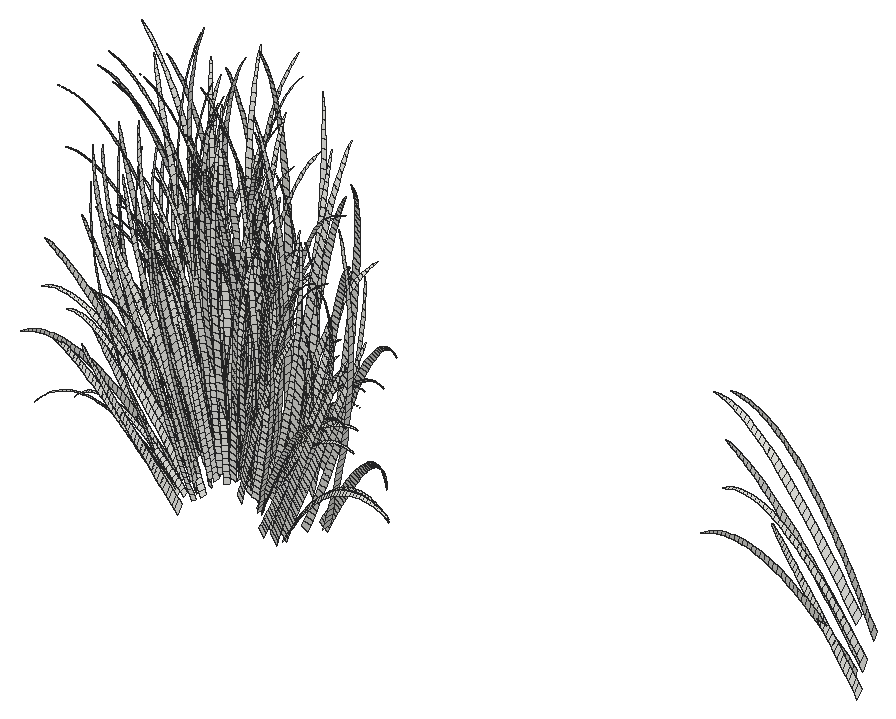
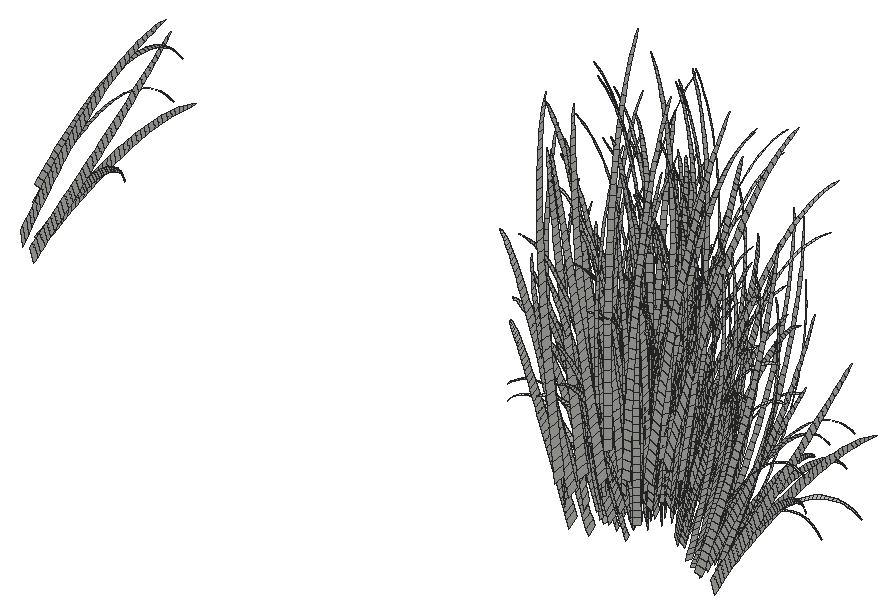
# SketchUp Ruby script. Lengths in inches.
U = 1.inch
M = Sketchup.active_model
def pt(a) = Geom::Point3d.new(a.map { |v| v * U })
def face(e, loops, mat)
  f = e.add_face(loops[0].map { |a| pt(a) })
  loops[1..].each { |l| e.add_face(l.map { |a| pt(a) }).erase! }
  f.material = f.back_material = mat if mat
  f
end
# faces: each face lists its corners as indices into pts; further lists are holes
def faces(e, pts, list, mat = nil) = list.each { |f| face(e, (f[0].is_a?(Array) ? f : [f]).map { |l| l.map { |i| pts[i] } }, mat) }
# xy, xz, yz: faces in a plane at the given z, y or x. An outline is a flat list of corners, or four numbers for a rectangle; further outlines are holes
def ring(l) = l.size == 4 ? [[l[0], l[1]], [l[2], l[1]], [l[2], l[3]], [l[0], l[3]]] : l.each_slice(2).to_a
def flat(e, list, mat, &to3) = list.each { |f| face(e, (f[0].is_a?(Array) ? f : [f]).map { |l| ring(l).map { |u, v| to3.(u, v) } }, mat) }
def xy(e, z, list, mat = nil) = flat(e, list, mat) { |x, y| [x, y, z] }
def xz(e, y, list, mat = nil) = flat(e, list, mat) { |x, z| [x, y, z] }
def yz(e, x, list, mat = nil) = flat(e, list, mat) { |y, z| [x, y, z] }
def lines(e, pts, list) = list.each { |a, b| e.add_line(pt(pts[a]), pt(pts[b])) }
# prism: a flat outline (further loops are holes) pulled along v
def prism(e, loops, v, mat = nil)
  f = face(e, loops, mat); d = Geom::Vector3d.new(v.map { |x| x * U })
  f.pushpull(f.normal.samedirection?(d) ? d.length : -d.length)
end
def box(e, o, s, mat = nil) = prism(e, [[o, [o[0] + s[0], o[1], o[2]], [o[0] + s[0], o[1] + s[1], o[2]], [o[0], o[1] + s[1], o[2]]]], [0, 0, s[2]], mat)
def at(x, y, z, deg = 0) = Geom::Transformation.translation(pt([x, y, z])) * Geom::Transformation.rotation(ORIGIN, Z_AXIS, deg.degrees)
def axes(o, x, y, z) = Geom::Transformation.new([*x, 0, *y, 0, *z, 0, *pt(o).to_a, 1])
def part(name) = M.definitions.add(name)
# library, detail: a bought-in or finely detailed component or shape, given as its bounding box
def library(name, o, s) = part(name).tap { |d| box(d.entities, o, s) }
def detail(e, o, s) = box(e.add_group.entities, o, s)
def put(e, d, t, mat = nil) = e.add_instance(d, t).tap { |i| i.material = mat if mat }
def group(e, t, mat = nil) = e.add_group.tap { |g| g.transformation = t; g.material = mat if mat }.entities
root = M.entities
c1 = part("fur_instance\#8")
p = [[-0.25,1.49,0.03],[0.25,-1.49,-0.03],[0.44,-1.47,1.51],[-0.05,1.47,1.57],[0.65,-1.44,3.05],[0.16,1.45,3.11],
  [0.86,-1.42,4.59],[0.38,1.44,4.65],[1.1,-1.39,6.13],[0.62,1.43,6.18],[1.34,-1.35,7.66],[0.875,1.42,7.72],
  [1.6,-1.32,9.19],[1.14,1.41,9.25],[1.88,-1.28,10.72],[1.43,1.41,10.78],[2.18,-1.24,12.25],[1.73,1.41,12.3],
  [2.49,-1.19,13.77],[2.05,1.41,13.82],[2.83,-1.15,15.29],[2.4,1.41,15.34],[3.18,-1.09,16.8],[2.76,1.42,16.85],
  [3.56,-1.03,18.31],[3.14,1.43,18.35],[3.96,-0.97,19.81],[3.55,1.44,19.85],[4.38,-0.91,21.3],[3.99,1.46,21.35],
  [4.84,-0.83,22.78],[4.45,1.48,22.83],[5.32,-0.76,24.26],[4.93,1.51,24.31],[5.82,-0.67,25.73],[5.45,1.54,25.77],
  [6.36,-0.59,27.18],[6,1.57,27.23],[6.93,-0.49,28.625],[6.58,1.61,28.67],[7.54,-0.39,30.05],[7.19,1.66,30.1],
  [8.18,-0.28,31.47],[7.84,1.71,31.51],[8.85,-0.16,32.86],[8.53,1.77,32.9],[9.57,-0.04,34.24],[9.25,1.83,34.27],
  [10.32,0.09,35.59],[10.02,1.9,35.625],[11.12,0.23,36.92],[10.82,1.97,36.95],[11.95,0.38,38.22],[11.67,2.06,38.25],
  [12.84,0.54,39.49],[12.57,2.14,39.52],[13.76,0.71,40.73],[13.51,2.24,40.76],[14.73,0.89,41.93],[14.49,2.34,41.95],
  [15.75,1.08,43.09],[15.52,2.45,43.11],[16.82,1.28,44.2],[16.6,2.5625,44.23],[17.93,1.5,45.27],[17.73,2.68,45.29],
  [19.08,1.73,46.28],[18.9,2.81,46.3],[20.29,1.97,47.24],[20.125,2.93,47.26],[21.53,2.22,48.13],[21.39,3.0625,48.15],
  [22.82,2.5,48.96],[22.7,3.1875,48.98],[24.14,2.8125,49.72],[24.06,3.3,49.73],[25.48,3.27,50.41]]
faces(c1.entities,p,[[0,1,2,3],[3,2,4,5],[5,4,6,7],[7,6,8,9],[9,8,10,11],[11,10,12,13],[13,12,14,15],[15,14,16,17],
  [17,16,18,19],[19,18,20,21],[21,20,22,23],[23,22,24,25],[25,24,26,27],[27,26,28,29],[29,28,30,31],[31,30,32,33],
  [33,32,34,35],[35,34,36,37],[37,36,38,39],[39,38,40,41],[41,40,42,43],[43,42,44,45],[45,44,46,47],[47,46,48,49],
  [49,48,50,51],[51,50,52,53],[53,52,54,55],[55,54,56,57],[57,56,58,59],[59,58,60,61],[61,60,62,63],[63,62,64,65],
  [65,64,66,67],[67,66,68,69],[69,68,70,71],[71,70,72,73],[73,72,74,75],[75,74,76]])
put(root,c1,axes([95.76,70.05,-3.04],[0.01897,-0.21218,0.0586],[0.13531,-0.01729,0.38322],[-0.17657,-0.01268,0.31544]))
put(root,c1,axes([96.34,68.3125,-2.78],[-0.03242,-0.16161,-0.19656],[0.13271,-0.12456,0.32589],[-0.17032,-0.04313,0.30667]))
put(root,c1,axes([97.72,67.32,-0.53],[-0.17146,0.07712,-0.27655],[0.00216,-0.17859,-0.14821],[-0.13359,-0.07259,0.37194]))
put(root,c1,axes([97.38,67.44,-3.66],[-0.07927,0.1771,-0.13212],[-0.09456,-0.05104,-0.31736],[-0.15384,-0.03896,0.27701]))
put(root,c1,axes([97.58,67.0625,-2.9],[-0.11039,-0.00414,-0.3495],[0.07669,-0.1786,0.00651],[-0.14786,-0.06719,0.2791]))
put(root,c1,axes([98.16,65.8125,-2.88],[-0.13594,0.15084,-0.11164],[-0.0609,-0.07291,-0.33491],[-0.13519,-0.09407,0.27953]))
put(root,c1,axes([95.88,69.58,-2.68],[0.13391,-0.00422,0.37894],[-0.02725,0.21287,-0.08205],[-0.17659,-0.01268,0.31548]))
put(root,c1,axes([98.56,66.53,-1.61],[-0.14992,0.10635,-0.20855],[-0.03569,-0.13875,-0.18978],[-0.12006,-0.06524,0.33426]))
put(root,c1,axes([98.55,67.96,-1.74],[-0.13947,0.07457,-0.26376],[-0.03048,-0.16347,-0.05841],[-0.12421,-0.01975,0.3263]))
put(root,c1,axes([98.58,66.7,-3.14],[-0.11214,0.07357,-0.29467],[-0.00419,-0.1506,-0.10442],[-0.13991,-0.03543,0.25192]))
put(root,c1,axes([97.64,70.26,4.84],[-0.16722,-0.14584,-0.14657],[0.18274,-0.19209,0.09427],[-0.0816,-0.06233,0.55718]))
put(root,c1,axes([96.18,71.21,-1.63],[0.10956,-0.18152,0.25882],[0.13509,0.11782,0.19082],[-0.14519,0.00192,0.39222]))
put(root,c1,axes([97.17,69.17,-2.25],[0.07012,-0.18381,0.20265],[0.10518,0.07075,0.29594],[-0.16336,-0.01173,0.29184]))
put(root,c1,axes([97.06,66.95,-2.91],[0.11177,0.01694,0.37048],[-0.08915,0.18926,-0.03147],[-0.15727,-0.07147,0.29687]))
put(root,c1,axes([97.58,67.58,-2.4],[0.07273,0.09595,0.27862],[-0.10249,0.16133,-0.212],[-0.15668,-0.03967,0.28211]))
put(root,c1,axes([96.1,68.47,-1.64],[0.16226,-0.13696,0.26442],[0.06401,0.16282,0.19515],[-0.14822,-0.05035,0.39313]))
put(root,c1,axes([98.9375,68.57,3.38],[-0.19486,-0.07064,-0.15993],[0.11436,-0.20339,0.01183],[-0.07048,-0.06892,0.50496]))
put(root,c1,axes([99.14,65.35,-3.56],[-0.09839,0.14314,-0.01192],[-0.08354,-0.02419,-0.30566],[-0.11714,-0.08151,0.24221]))
put(root,c1,axes([98.54,68.2,-3.06],[-0.01321,-0.17005,0.06481],[0.1141,-0.02557,0.30569],[-0.13946,0.01456,0.25678]))
put(root,c1,axes([99.65,69.16,1.2],[-0.18243,0.01895,-0.19563],[-0.00133,-0.1948,0.08688],[-0.09334,0.00298,0.40574]))
put(root,c1,axes([99.52,67.88,-0.75],[-0.16023,0.03354,-0.19126],[-0.00898,-0.17162,0.02853],[-0.08895,-0.01176,0.36236]))
put(root,c1,axes([99.47,66.625,0.58],[-0.1494,0.14445,-0.05993],[-0.10862,-0.10225,-0.21391],[-0.08642,-0.08137,0.39881]))
put(root,c1,axes([96.96,68.125,-0.75],[0.16036,-0.12824,0.26431],[0.05712,0.1633,0.18167],[-0.14465,-0.04914,0.38366]))
put(root,c1,axes([97.38,68.18,-1.53],[0.12489,0.06673,0.27563],[-0.09958,0.18305,-0.12082],[-0.13573,-0.04611,0.36]))
put(root,c1,axes([99.77,66.73,-0.91],[-0.15052,-0.00251,-0.18515],[0.03159,-0.16716,0.03488],[-0.08794,-0.02622,0.34898]))
put(root,c1,axes([99.5,68.69,-0.2],[-0.10618,-0.13262,-0.04878],[0.13367,-0.1263,0.19427],[-0.08735,0.00279,0.37967]))
put(root,c1,axes([98.35,68.18,-3.57],[0.10833,0.05099,0.24664],[-0.03776,0.16401,-0.19126],[-0.1393,0.01454,0.25647]))
put(root,c1,axes([99.47,70.78,6.02],[-0.09372,-0.20637,-0.07363],[0.22677,-0.12712,0.15354],[-0.08199,-0.04812,0.55353]))
put(root,c1,axes([97.89,69.19,-1.1],[0.15491,-0.05585,0.29054],[0.02871,0.18789,-0.02061],[-0.13151,0.00174,0.35528]))
put(root,c1,axes([100.5,67.92,0.34],[-0.13836,0.10656,-0.19014],[-0.08729,-0.13946,-0.02631],[-0.08371,0.00267,0.36384]))
put(root,c1,axes([99.375,66.87,-1.86],[0.03066,0.14936,0.05869],[-0.12804,0.07175,-0.24213],[-0.11455,-0.01821,0.30092]))
put(root,c1,axes([99.75,66.9375,2.03],[-0.03053,0.18634,0.11663],[-0.19498,0.03215,-0.20672],[-0.09234,-0.08694,0.42611]))
put(root,c1,axes([99.99,66.09,0.62],[-0.076,0.1669,0.09562],[-0.17144,-0.01335,-0.19918],[-0.07397,-0.09509,0.39348]))
put(root,c1,axes([100.3125,67.9,0.96],[-0.14595,-0.08896,-0.08701],[0.11069,-0.159,0.08949],[-0.05969,-0.02587,0.41282]))
put(root,c1,axes([100.32,66.87,1.13],[-0.13003,0.1505,-0.04051],[-0.13515,-0.09639,-0.12681],[-0.0585,-0.05721,0.41915]))
put(root,c1,axes([100.31,69.73,4.93],[-0.20007,-0.1011,-0.05198],[0.13259,-0.20105,0.02025],[-0.03025,-0.05245,0.53866]))
put(root,c1,axes([100.8125,69.61,6.05],[-0.23914,-0.05106,-0.06078],[0.08551,-0.22855,-0.0252],[-0.02809,-0.06875,0.5682]))
put(root,c1,axes([99.25,67.93,-3.57],[0.06974,-0.11239,0.27242],[0.09117,0.10684,0.0892],[-0.12045,0.03482,0.23783]))
put(root,c1,axes([98.43,69.49,-1.98],[0.12819,-0.10555,0.27193],[0.08655,0.15023,0.02614],[-0.11644,0.02211,0.33646]))
put(root,c1,axes([99.42,66.64,-3.27],[0.09888,-0.02928,0.28041],[-0.00291,0.15131,-0.01175],[-0.12783,-0.00918,0.22836]))
put(root,c1,axes([99.94,68.41,-1.64],[-0.01787,-0.16163,0.13786],[0.14541,-0.01364,0.20157],[-0.09392,0.03632,0.30351]))
put(root,c1,axes([100.86,66.9,0.16],[-0.15295,0.08658,-0.10984],[-0.06653,-0.14152,-0.02919],[-0.05435,-0.02356,0.3759]))
put(root,c1,axes([100.52,68.36,-1.61],[-0.08732,-0.12975,0.07004],[0.12156,-0.08169,0.22443],[-0.07712,0.04857,0.29461]))
put(root,c1,axes([101.34,69.47,6.1],[-0.24023,0.10194,-0.01182],[-0.08393,-0.20819,-0.06775],[-0.02132,-0.07588,0.56748]))
put(root,c1,axes([99.06,66.95,-1.92],[0.13512,-0.04534,0.25565],[0.00767,0.16418,0.01521],[-0.11775,-0.01872,0.30933]))
put(root,c1,axes([101.21,66.88,0.11],[-0.16155,0.04363,-0.11105],[-0.02173,-0.15615,0.00187],[-0.05311,-0.02302,0.36735]))
put(root,c1,axes([101.125,68.14,0.01],[-0.13763,-0.08778,-0.02445],[0.09224,-0.14199,0.18002],[-0.06167,0.02548,0.35158]))
put(root,c1,axes([100.82,67.91,4.45],[-0.11071,0.19643,0.08485],[-0.20741,-0.05916,-0.14436],[-0.04649,-0.10158,0.50968]))
put(root,c1,axes([99.14,67.375,0.375],[0.12398,0.09622,0.18511],[-0.12468,0.16008,-0.11198],[-0.09878,-0.04719,0.39625]))
put(root,c1,axes([101.45,67.29,0.93],[-0.15275,-0.06369,-0.07605],[0.08272,-0.1606,0.08732],[-0.05298,-0.01559,0.38969]))
put(root,c1,axes([101.29,66.44,0.1],[-0.12167,0.12231,-0.08026],[-0.10576,-0.10199,-0.07795],[-0.05387,-0.03162,0.36369]))
put(root,c1,axes([99.79,67.73,0.52],[0.1073,0.11537,0.13468],[-0.12896,0.14123,-0.15523],[-0.09593,-0.0286,0.38067]))
put(root,c1,axes([101.6875,66.98,-0.06],[-0.15222,0.06371,-0.10078],[-0.04912,-0.14483,0.02613],[-0.04368,-0.00705,0.35627]))
put(root,c1,axes([101.84,66.57,1.76],[-0.18454,0.07316,-0.01839],[-0.05778,-0.16138,-0.04792],[-0.01906,-0.05522,0.43193]))
put(root,c1,axes([100.54,71.5625,4.7],[-0.03022,-0.22611,0.09029],[0.23429,-0.05028,0.11994],[-0.05481,-0.00145,0.5217]))
put(root,c1,axes([100.03,65.9,0.83],[0.08886,0.11953,0.22309],[-0.17307,0.12603,-0.0526],[-0.07674,-0.09865,0.40821]))
put(root,c1,axes([101.95,69.69,5.24],[-0.19122,-0.11806,-0.01455],[0.14538,-0.19433,0.04316],[-0.02276,-0.03764,0.53822]))
put(root,c1,axes([100.95,68.76,1.41],[-0.07059,-0.16734,0.04684],[0.17777,-0.08469,0.11217],[-0.04438,-0.00118,0.42241]))
put(root,c1,axes([102.04,67.4,0.8],[-0.1632,-0.04584,-0.02491],[0.06111,-0.16287,0.10545],[-0.03205,0.00396,0.38155]))
put(root,c1,axes([101.26,67.78,0.43],[-0.07809,-0.14325,0.0107],[0.15359,-0.09235,0.11164],[-0.04706,-0.00759,0.38378]))
put(root,c1,axes([102.12,68.24,1.7],[-0.18597,0.0618,-0.02273],[-0.04748,-0.17087,0.02426],[-0.01189,-0.02692,0.4292]))
put(root,c1,axes([100.38,67.35,-2.1],[0.12505,0.02128,0.17693],[-0.02026,0.14885,-0.13694],[-0.09536,0.01811,0.27556]))
put(root,c1,axes([98.5,70.37,4.92],[0.23978,-0.07082,0.15768],[0.03022,0.22441,0.06362],[-0.07961,-0.06081,0.54364]))
put(root,c1,axes([101.25,68.31,3.06],[-0.04674,0.1979,-0.00041],[-0.20698,-0.02041,-0.04932],[-0.02674,-0.04637,0.47621]))
put(root,c1,axes([98.9,68.09,4.41],[0.21026,0.07749,0.17035],[-0.13208,0.20951,0.0486],[-0.06062,-0.09852,0.54406]))
put(root,c1,axes([99.26,69.1,2.46],[0.19711,0.03834,0.13931],[-0.07116,0.20343,-0.04176],[-0.07003,-0.0411,0.47276]))
put(root,c1,axes([100.61,67.91,-0.74],[0.08378,-0.14307,0.16626],[0.13275,0.07958,0.06416],[-0.07048,0.0146,0.34149]))
put(root,c1,axes([102.4,65.47,-0.05],[-0.14611,0.07417,-0.01085],[-0.0636,-0.12579,-0.04088],[-0.01571,-0.04551,0.35595]))
put(root,c1,axes([101.92,65.52,-0.11],[-0.03907,0.14419,0.04289],[-0.15068,-0.00691,-0.10234],[-0.04404,-0.05511,0.34471]))
put(root,c1,axes([102.72,66.39,1.99],[-0.18895,0.06999,0.02245],[-0.05996,-0.16418,-0.04942],[-0.00199,-0.06326,0.44045]))
put(root,c1,axes([101.76,68.33,4.43],[-0.07149,0.20688,0.05021],[-0.22153,-0.04139,-0.03916],[-0.01557,-0.07173,0.51835]))
put(root,c1,axes([102.36,67.78,-0.98],[-0.12985,-0.07677,0.07158],[0.09092,-0.12597,0.14453],[-0.01646,0.03757,0.31821]))
put(root,c1,axes([101.85,66.36,0.1],[0.0007,0.15498,-0.03624],[-0.15701,0.01919,-0.0982],[-0.04789,-0.01409,0.35225]))
put(root,c1,axes([99.64,69.85,3.34],[0.21533,-0.00022,0.14201],[-0.02985,0.21622,-0.04212],[-0.07083,-0.0307,0.48991]))
put(root,c1,axes([101.76,69.9,1.31],[-0.05762,-0.17661,0.09378],[0.18885,-0.07013,0.07584],[-0.02585,0.00825,0.42914]))
put(root,c1,axes([102.47,66.12,1.29],[-0.11204,0.14362,0.03398],[-0.14775,-0.08605,-0.03808],[-0.00899,-0.05843,0.41243]))
put(root,c1,axes([101.42,66.88,0.34],[0.07256,0.13813,0.01061],[-0.14853,0.08916,-0.10968],[-0.05042,-0.01484,0.37084]))
put(root,c1,axes([103.28,68.28,2.5],[-0.20122,0.04978,0.02765],[-0.03696,-0.18587,0.02525],[0.00919,-0.0352,0.4569]))
put(root,c1,axes([102.08,69.16,2.61],[-0.07053,-0.17965,0.10788],[0.19435,-0.08267,0.06265],[-0.01549,0.01046,0.44704]))
put(root,c1,axes([102.6875,67,0.08],[-0.12044,0.11617,-0.06507],[-0.11184,-0.10532,0.07409],[-0.00291,0.00808,0.35453]))
put(root,c1,axes([101.09,66.82,1.47],[0.1306,0.09776,0.12408],[-0.13059,0.14634,-0.04229],[-0.05761,-0.05634,0.41276]))
put(root,c1,axes([102.94,67,0.32],[-0.14146,0.09732,-0.03277],[-0.08974,-0.12702,0.09515],[0.00654,0.00629,0.36155]))
put(root,c1,axes([102.26,66.14,1.84],[-0.02865,0.1632,0.13083],[-0.19416,0.00105,-0.04665],[-0.01776,-0.09378,0.4187]))
put(root,c1,axes([100.21,68.21,3.96],[0.21896,0.00722,0.14738],[-0.05367,0.20894,0.06409],[-0.06377,-0.07981,0.49923]))
put(root,c1,axes([102.14,66.79,0.41],[-0.005,0.15882,-0.01867],[-0.16818,0.01184,-0.02587],[-0.01594,-0.02637,0.37698]))
put(root,c1,axes([103.12,68.37,-1.29],[-0.15178,-0.03817,0.09021],[0.05761,-0.14672,0.13772],[0.01323,0.03497,0.32535]))
put(root,c1,axes([103.09,68.04,-0.72],[-0.14817,-0.05096,0.10268],[0.07099,-0.14472,0.13123],[0.01339,0.03539,0.32926]))
put(root,c1,axes([102.65,65.7,0.44],[-0.04364,0.1509,0.04181],[-0.16335,-0.02313,-0.02043],[-0.0082,-0.05328,0.37608]))
put(root,c1,axes([101.25,66.81,1.18],[0.16328,0.03799,0.12354],[-0.06943,0.16853,-0.0179],[-0.05845,-0.04464,0.39911]))
put(root,c1,axes([102.84,68.17,0.11],[-0.0829,-0.13844,0.09301],[0.15279,-0.09132,0.04718],[-0.00308,0.00854,0.37496]))
put(root,c1,axes([101.38,68.7,1.45],[0.11915,-0.15444,0.11959],[0.14734,0.10329,0.01409],[-0.04397,-0.00116,0.41847]))
put(root,c1,axes([100.86,68.36,1.08],[0.18469,-0.02182,0.1026],[0.00322,0.18141,-0.06268],[-0.05045,-0.00814,0.41143]))
put(root,c1,axes([102.97,67.02,3.23],[-0.06667,0.19226,0.05915],[-0.20819,-0.04319,-0.00198],[0.00188,-0.06909,0.48578]))
put(root,c1,axes([103.09,68.83,0.96],[-0.10911,-0.1372,0.1051],[0.15387,-0.1168,0.04236],[0.00736,0.00708,0.40712]))
put(root,c1,axes([101.51,66.2,-0.03],[0.15146,0.01629,0.10652],[-0.04117,0.15418,-0.02273],[-0.05245,-0.03078,0.35407]))
put(root,c1,axes([102.23,69.19,1.46],[0.00836,-0.18662,0.11674],[0.19508,-0.00753,0.01588],[-0.01463,0.00988,0.4222]))
put(root,c1,axes([101.2,68.6,2.83],[0.12224,-0.1724,0.03147],[0.17004,0.09672,0.03094],[-0.02457,-0.03858,0.46994]))
put(root,c1,axes([102.42,71.77,4.23],[-0.01914,-0.22341,0.14227],[0.23668,-0.03758,0.00754],[-0.0042,0.01167,0.5122]))
put(root,c1,axes([103.37,65.51,-0.04],[-0.08483,0.12977,0.03637],[-0.13576,-0.06868,0.01436],[0.01015,-0.0438,0.35695]))
put(root,c1,axes([101.62,66.92,1.63],[0.13112,0.1119,0.04642],[-0.13781,0.13647,-0.01148],[-0.02271,-0.04835,0.42618]))
put(root,c1,axes([100.73,67.25,3.98],[0.22597,0.02863,0.10796],[-0.07525,0.20019,0.13019],[-0.03474,-0.10937,0.51158]))
put(root,c1,axes([103.58,70.6,2.2],[-0.12335,-0.15584,0.12717],[0.17408,-0.13265,0.02266],[0.01997,0.00343,0.46197]))
put(root,c1,axes([102.85,68.51,2.56],[-0.03248,-0.18789,0.03246],[0.20264,-0.04691,-0.01246],[0.00277,-0.0305,0.45814]))
put(root,c1,axes([102.25,70.71,0.1],[0.06236,-0.17527,0.19539],[0.18475,0.04701,-0.03446],[-0.02024,0.04621,0.39144]))
put(root,c1,axes([100.37,70.18,6.02],[0.24246,-0.09581,0.04741],[0.07374,0.21618,0.03906],[-0.03158,-0.05994,0.56838]))
put(root,c1,axes([102.6,69.22,2.74],[0.00458,-0.19714,0.03462],[0.20895,-0.01368,-0.00104],[-0.00501,-0.02872,0.46671]))
put(root,c1,axes([102.06,66.2,3.59],[0.08928,0.17665,0.16183],[-0.22737,0.09539,0.05927],[-0.00818,-0.11915,0.51927]))
put(root,c1,axes([101.54,68.33,0.25],[0.167,0.03821,0.03014],[-0.05354,0.16593,-0.1048],[-0.03226,0.00399,0.38398]))
put(root,c1,axes([103.84,67.23,-0.4],[-0.11227,0.12169,-0.01571],[-0.11695,-0.0983,0.09825],[0.0234,-0.00238,0.35291]))
put(root,c1,axes([103.32,68.5,5.09],[-0.01737,0.2214,0.05487],[-0.24332,0.00145,0.03189],[0.01003,-0.07326,0.54284]))
put(root,c1,axes([103.07,65.79,2.0625],[-0.01068,0.1751,0.14296],[-0.21108,0.00073,0.04004],[0.01667,-0.10172,0.45077]))
put(root,c1,axes([103.55,68.3,2.77],[-0.03706,0.19452,0.0025],[-0.2058,-0.02021,0.04233],[0.01369,-0.04269,0.4672]))
put(root,c1,axes([103.08,67.62,2.76],[0.00321,0.19067,0.02092],[-0.20749,0.01649,0.04397],[0.01444,-0.0534,0.46311]))
put(root,c1,axes([102.91,66.97,0.65],[0.0444,0.15353,-0.02873],[-0.16709,0.05572,0.00025],[-0.00083,-0.02443,0.38596]))
put(root,c1,axes([101.54,67.77,2.05],[0.19137,0.02245,0.03812],[-0.04546,0.1843,-0.01629],[-0.02307,-0.03624,0.44138]))
put(root,c1,axes([102.57,69.2,3.94],[0.0752,-0.20516,0.02464],[0.21175,0.0536,-0.02901],[0.00304,-0.03339,0.50163]))
put(root,c1,axes([102.39,70.36,-0.02],[0.1059,-0.15637,0.15831],[0.16025,0.08485,-0.11228],[-0.00207,0.04487,0.3837]))
put(root,c1,axes([104.78,69.14,4.55],[-0.20879,-0.09834,0.1321],[0.10662,-0.20129,-0.08744],[0.06463,-0.06137,0.52082]))
put(root,c1,axes([103.11,67.43,0.59],[0.04623,0.15623,-0.10375],[-0.16763,0.05842,0.01792],[0.01628,0.0028,0.37652]))
put(root,c1,axes([102.39,66.62,0.47],[0.15712,0.04243,0.01115],[-0.06087,0.1538,-0.0283],[-0.01337,-0.02475,0.37716]))
put(root,c1,axes([103.58,67.09,0.04],[-0.02615,-0.15514,0.08978],[0.1636,-0.03862,-0.04775],[0.02391,-0.00243,0.36067]))
put(root,c1,axes([102.29,68.37,-0.01],[0.17226,-0.02677,0.04434],[0.01787,0.15893,-0.17055],[-0.01798,0.04104,0.34767]))
put(root,c1,axes([102.1875,69.57,2.49],[0.17834,-0.11625,0.08266],[0.1071,0.16149,-0.09447],[-0.01558,0.01053,0.44981]))
put(root,c1,axes([104.96,67.0625,1.62],[-0.15292,0.11854,0.12624],[-0.12574,-0.14279,0.04956],[0.05301,-0.06232,0.4383]))
put(root,c1,axes([104.2,68.91,-0.45],[-0.09023,-0.13424,0.18354],[0.14991,-0.10591,-0.00994],[0.04513,0.02354,0.36032]))
put(root,c1,axes([103.76,66.69,-0.04],[0.01188,0.15545,-0.07184],[-0.16156,0.0237,0.07132],[0.03067,-0.00873,0.35494]))
put(root,c1,axes([103.7,65.76,0.375],[-0.00201,0.1516,0.05729],[-0.16575,-0.0022,0.09935],[0.04109,-0.06021,0.3647]))
put(root,c1,axes([105.09,67.33,-1.04],[-0.15312,0.05179,0.12153],[-0.03636,-0.15379,0.12597],[0.06399,-0.0008,0.33763]))
put(root,c1,axes([103.11,66.54,0.25],[0.13491,0.07893,-0.02845],[-0.09527,0.13412,-0.00523],[0.005,-0.02625,0.36875]))
put(root,c1,axes([103.83,69.04,-0.53],[0.00974,-0.16765,0.16266],[0.17627,-0.01134,-0.08044],[0.03031,0.03221,0.35757]))
put(root,c1,axes([104.67,66.65,-0.37],[-0.12808,-0.08127,0.17105],[0.08472,-0.13879,-0.03962],[0.07069,-0.01437,0.33524]))
put(root,c1,axes([103.77,72.16,6.37],[-0.01557,-0.2472,0.11257],[0.25666,-0.03446,-0.11464],[0.04868,-0.01385,0.56337]))
put(root,c1,axes([102.99,68.8,5.83],[0.1638,0.16225,0.02835],[-0.19372,0.16204,0.06129],[0.00656,-0.07857,0.56406]))
put(root,c1,axes([103.5,67.81,-1.125],[0.06075,-0.14439,0.11282],[0.14535,0.04045,-0.11615],[0.02704,0.02874,0.31908]))
put(root,c1,axes([103.9,67.84,3.67],[0.00546,0.20018,0.07075],[-0.21886,0.00452,0.13393],[0.05427,-0.07952,0.48166]))
put(root,c1,axes([102.96,69.05,3.53],[0.1489,-0.1631,0.00196],[0.16131,0.12724,-0.0384],[0.00665,-0.0349,0.49014]))
put(root,c1,axes([105.52,68.03,0.43],[-0.17727,-0.00884,0.19718],[0.01815,-0.18643,0.05134],[0.08203,-0.01667,0.38902]))
put(root,c1,axes([102.47,68.81,5.07],[0.24085,-0.01288,-0.01594],[-0.00713,0.21681,0.06326],[0.00207,-0.07616,0.53545]))
put(root,c1,axes([105.6,68.4,2.07],[-0.19467,0.01004,0.22404],[-0.00781,-0.20399,0.04036],[0.09618,-0.03688,0.42982]))
put(root,c1,axes([102.48,69.48,6.18],[0.24462,0.04853,-0.00958],[-0.07419,0.22591,0.06737],[0.00661,-0.07917,0.56836]))
put(root,c1,axes([103.24,67.41,0.375],[0.16085,-0.07091,-0.00868],[0.05991,0.14859,-0.10356],[0.01607,0.00276,0.37166]))
put(root,c1,axes([105.22,66.49,-1.07],[-0.09933,0.11915,0.09682],[-0.11277,-0.10305,0.14649],[0.07419,-0.02845,0.33155]))
put(root,c1,axes([103.96,65.87,2.15],[0.1142,0.15271,0.07486],[-0.18421,0.10064,0.13224],[0.02836,-0.10071,0.46512]))
put(root,c1,axes([104.38,66.91,-1.12],[0.01848,-0.15029,0.09797],[0.14831,0.00119,-0.12824],[0.05045,0.01072,0.31409]))
put(root,c1,axes([103.1,67.96,3.62],[0.21441,0.03504,-0.02755],[-0.05444,0.19871,0.04867],[0.01191,-0.06374,0.49276]))
put(root,c1,axes([103.61,66.59,-0.12],[0.15483,0.02452,-0.08835],[-0.03742,0.15266,-0.04583],[0.03016,-0.00858,0.34899]))
put(root,c1,axes([104.1,66.39,-0.44],[0.12172,0.08749,-0.09823],[-0.09805,0.12464,0.01693],[0.03543,-0.01566,0.34464]))
put(root,c1,axes([105.64,70.26,1.11],[-0.10531,-0.16415,0.20039],[0.16955,-0.12413,-0.09552],[0.08116,-0.00102,0.4282]))
put(root,c1,axes([103.65,67.3,1.28],[0.15584,0.0797,-0.11547],[-0.0923,0.15744,0.00315],[0.04105,-0.01815,0.39937]))
put(root,c1,axes([106.7,68.26,2.19],[-0.20296,0.04396,0.25147],[-0.06114,-0.20583,-0.00189],[0.10319,-0.08007,0.46398]))
put(root,c1,axes([105.42,66.9,0.03],[-0.05241,0.16147,0.07727],[-0.15892,-0.06034,0.18232],[0.08415,-0.0479,0.3696]))
put(root,c1,axes([104.375,66.85,0.53],[0.10935,0.12723,-0.0806],[-0.13524,0.11022,0.08276],[0.04716,-0.03593,0.38648]))
put(root,c1,axes([105.89,66.15,-1.73],[-0.13363,0.01209,0.24348],[-0.02341,-0.15821,0.02454],[0.10585,-0.04288,0.29749]))
put(root,c1,axes([104.59,65.54,-0.89],[0.04868,0.13833,-0.04452],[-0.13249,0.04478,0.16098],[0.07098,-0.0404,0.31175]))
put(root,c1,axes([104.05,68.62,-1.45],[0.15705,-0.06817,-0.01855],[0.04537,0.13415,-0.23216],[0.04015,0.05663,0.29621]))
put(root,c1,axes([105.15,66.96,-1.66],[-0.0035,0.15221,-0.13037],[-0.13811,0.0204,0.18439],[0.08356,0.01425,0.28222]))
put(root,c1,axes([104.11,68.01,4.3],[0.18476,0.1259,-0.03463],[-0.14125,0.16417,0.15823],[0.05053,-0.09421,0.50755]))
put(root,c1,axes([106.17,67.04,-0.85],[-0.105,0.10997,0.20265],[-0.1047,-0.1341,0.17455],[0.11569,-0.04687,0.32514]))
put(root,c1,axes([104.37,68.72,1.53],[0.18917,-0.06704,-0.06686],[0.05451,0.17895,-0.10326],[0.03727,-0.0106,0.43133]))
put(root,c1,axes([105.71,67.5,-3.62],[-0.02967,-0.12807,0.22483],[0.11753,-0.07372,-0.14887],[0.10049,0.02798,0.22698]))
put(root,c1,axes([103.96,69.07,3.55],[0.21551,0.00607,-0.13742],[-0.0172,0.21045,-0.03067],[0.05502,-0.03283,0.47913]))
put(root,c1,axes([104.44,67.71,1.55],[0.18544,-0.04972,-0.1199],[0.04511,0.1779,-0.04118],[0.05175,-0.03943,0.42412]))
put(root,c1,axes([107.28,69.2,2.63],[-0.13857,0.17143,0.18015],[-0.17196,-0.14956,0.18932],[0.11106,-0.06322,0.48777]))
put(root,c1,axes([106.61,69.35,-1.51],[-0.08271,-0.14836,0.25336],[0.14839,-0.11682,-0.11362],[0.10275,0.01753,0.34702]))
put(root,c1,axes([104.89,67.73,-1.83],[0.1392,0.01865,-0.19659],[-0.04604,0.15192,-0.11441],[0.07206,0.03039,0.28637]))
put(root,c1,axes([104.54,69.6875,3.54],[0.2045,-0.09371,-0.11076],[0.08595,0.19464,-0.09275],[0.05645,-0.03369,0.4916]))
put(root,c1,axes([105.02,71.22,2.95],[0.13505,-0.18869,0.02697],[0.17317,0.11473,-0.23558],[0.07413,0.01575,0.4615]))
put(root,c1,axes([107.1,68.18,1.5],[-0.05009,0.1972,0.12811],[-0.20341,-0.06615,0.21296],[0.10198,-0.07913,0.45854]))
put(root,c1,axes([106.68,67.67,-1.2],[-0.05226,0.17384,0.04608],[-0.14605,-0.06174,0.27189],[0.11826,-0.02606,0.33853]))
put(root,c1,axes([106.25,65.9375,-3.28],[-0.0259,0.13847,0.08839],[-0.10293,-0.05886,0.26708],[0.12297,-0.03787,0.2304]))
put(root,c1,axes([105.15,67.41,1.34],[0.19428,0.00099,-0.13011],[-0.00447,0.1857,0.01775],[0.05358,-0.05088,0.43173]))
put(root,c1,axes([106.48,67.67,-3.03],[-0.0586,-0.13145,0.25194],[0.10919,-0.10295,-0.16429],[0.12358,0.00811,0.25105]))
put(root,c1,axes([105.39,66.77,-2.0625],[0.11365,-0.08796,-0.13302],[0.06535,0.12495,-0.18142],[0.09174,-0.00314,0.27875]))
put(root,c1,axes([105.91,68.98,-1.53],[0.12182,-0.13641,-0.05722],[0.10481,0.11532,-0.25636],[0.0972,0.01658,0.32827]))
put(root,c1,axes([105.66,68.15,-0.94],[0.15112,-0.07348,-0.15621],[0.04279,0.15836,-0.20373],[0.095,0.01621,0.32084]))
put(root,c1,axes([107.36,67.97,2.41],[0.03711,0.21617,0.09276],[-0.22705,0.0107,0.25479],[0.10293,-0.10542,0.49477]))
put(root,c1,axes([106.65,68.18,0.67],[0.10459,0.17012,-0.10766],[-0.16118,0.10117,0.20027],[0.09662,-0.055,0.42437]))
put(root,c1,axes([108.18,68.55,-3.39],[-0.11534,0.10838,0.24896],[-0.07338,-0.1624,0.25205],[0.15325,-0.01897,0.29298]))
put(root,c1,axes([106.17,66.17,-1.55],[0.13705,0.06092,-0.24143],[-0.03897,0.15511,0.08813],[0.11117,-0.04504,0.31244]))
put(root,c1,axes([107.88,69.52,-0.81],[-0.04683,-0.20253,0.13494],[0.1704,-0.05617,-0.28372],[0.13472,-0.02969,0.38568]))
put(root,c1,axes([106.4375,66.62,-2.14],[0.14053,0.00256,-0.25431],[0.0115,0.16488,-0.00221],[0.11001,-0.04457,0.30917]))
put(root,c1,axes([106.67,67.55,-1.81],[0.11573,-0.11352,-0.17299],[0.09518,0.13737,-0.20258],[0.11423,-0.02517,0.32701]))
put(root,c1,axes([107.51,65.75,-3.3],[0.04443,0.16095,0.1082],[-0.13761,-0.02397,0.33152],[0.13789,-0.09974,0.2801]))
put(root,c1,axes([108.04,72.45,2.57],[0.03522,-0.24577,0.05534],[0.23308,0.0235,-0.26379],[0.10852,-0.02206,0.51462]))
put(root,c1,axes([107.84,66.45,-3.17],[0.00679,0.17207,0.10989],[-0.13694,-0.04896,0.33579],[0.14998,-0.07528,0.28652]))
put(root,c1,axes([107.55,70.35,2.0625],[0.1074,-0.20139,-0.09354],[0.19115,0.11076,-0.2385],[0.10824,-0.04151,0.48371]))
put(root,c1,axes([106.9,69.12,-0.77],[0.15027,-0.10781,-0.18095],[0.0791,0.16599,-0.22838],[0.11882,-0.00407,0.36105]))
put(root,c1,axes([110.1,68.63,-2.63],[-0.15284,0.01805,0.42901],[-0.06641,-0.2167,0.01891],[0.18229,-0.0915,0.34824]))
put(root,c1,axes([107.78,67.28,-3.12],[0.12633,-0.01434,-0.33979],[0.03003,0.18353,-0.05493],[0.15045,-0.04633,0.28189]))
put(root,c1,axes([108.01,66.42,-3.25],[0.13942,0.04831,-0.34302],[0.00816,0.17572,0.1089],[0.15278,-0.07668,0.29185]))
put(root,c1,axes([108.26,70.61,0.6],[0.12813,-0.17071,-0.17976],[0.14324,0.15198,-0.29056],[0.14651,-0.03228,0.41943]))
put(root,c1,axes([109.53,69.0625,-3],[0.07286,-0.17069,-0.21842],[0.13329,0.1313,-0.33824],[0.176,-0.05419,0.32974]))
put(root,c1,axes([159.54,68.45,7.11],[-0.18691,0.1568,-0.23935],[-0.06787,-0.16218,-0.27405],[-0.15492,-0.08418,0.43132]))
put(root,c1,axes([158.78,71.27,4.24],[-0.09014,-0.18111,-0.08882],[0.15594,-0.13199,0.32093],[-0.15035,0.00199,0.40617]))
put(root,c1,axes([158.8125,70.05,2.34],[0.01897,-0.21218,0.0586],[0.13531,-0.01729,0.38322],[-0.17657,-0.01268,0.31544]))
put(root,c1,axes([159.39,68.3125,2.6],[-0.03242,-0.16161,-0.19656],[0.13271,-0.12456,0.32589],[-0.17032,-0.04313,0.30667]))
put(root,c1,axes([160.77,67.32,4.85],[-0.17146,0.07712,-0.27655],[0.00216,-0.17859,-0.14821],[-0.13359,-0.07259,0.37194]))
put(root,c1,axes([160.43,67.44,1.72],[-0.07927,0.1771,-0.13212],[-0.09456,-0.05104,-0.31736],[-0.15384,-0.03896,0.27701]))
